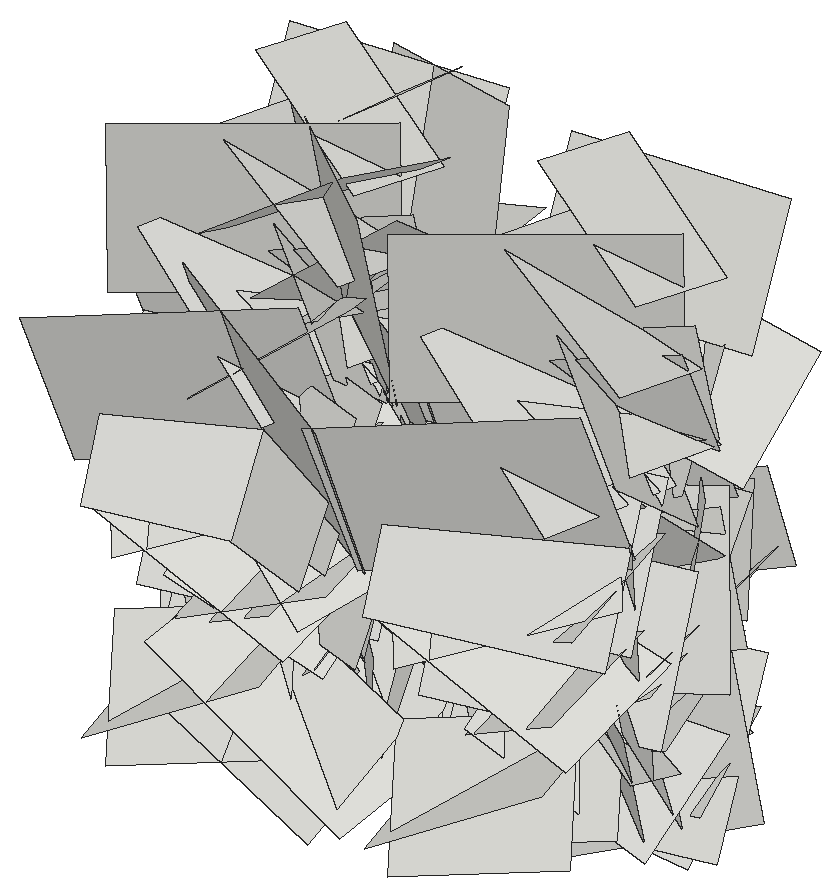
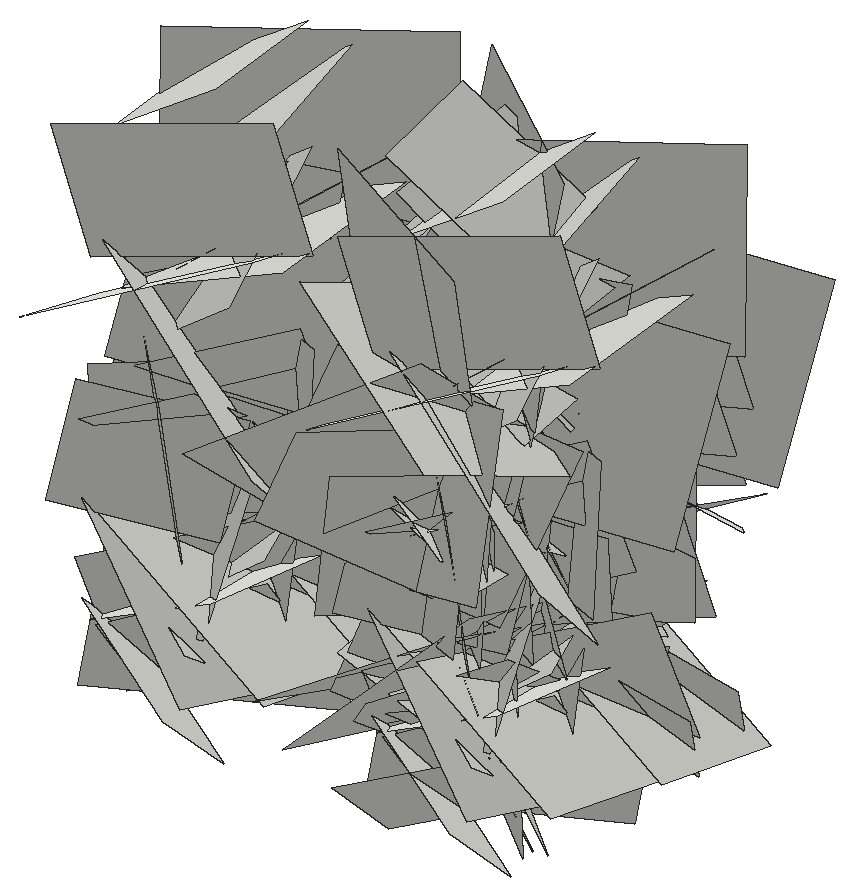
# SketchUp Ruby script. Lengths in inches.
U = 1.inch
M = Sketchup.active_model
def pt(a) = Geom::Point3d.new(a.map { |v| v * U })
def face(e, loops, mat)
  f = e.add_face(loops[0].map { |a| pt(a) })
  loops[1..].each { |l| e.add_face(l.map { |a| pt(a) }).erase! }
  f.material = f.back_material = mat if mat
  f
end
# faces: each face lists its corners as indices into pts; further lists are holes
def faces(e, pts, list, mat = nil) = list.each { |f| face(e, (f[0].is_a?(Array) ? f : [f]).map { |l| l.map { |i| pts[i] } }, mat) }
# xy, xz, yz: faces in a plane at the given z, y or x. An outline is a flat list of corners, or four numbers for a rectangle; further outlines are holes
def ring(l) = l.size == 4 ? [[l[0], l[1]], [l[2], l[1]], [l[2], l[3]], [l[0], l[3]]] : l.each_slice(2).to_a
def flat(e, list, mat, &to3) = list.each { |f| face(e, (f[0].is_a?(Array) ? f : [f]).map { |l| ring(l).map { |u, v| to3.(u, v) } }, mat) }
def xy(e, z, list, mat = nil) = flat(e, list, mat) { |x, y| [x, y, z] }
def xz(e, y, list, mat = nil) = flat(e, list, mat) { |x, z| [x, y, z] }
def yz(e, x, list, mat = nil) = flat(e, list, mat) { |y, z| [x, y, z] }
def lines(e, pts, list) = list.each { |a, b| e.add_line(pt(pts[a]), pt(pts[b])) }
# prism: a flat outline (further loops are holes) pulled along v
def prism(e, loops, v, mat = nil)
  f = face(e, loops, mat); d = Geom::Vector3d.new(v.map { |x| x * U })
  f.pushpull(f.normal.samedirection?(d) ? d.length : -d.length)
end
def box(e, o, s, mat = nil) = prism(e, [[o, [o[0] + s[0], o[1], o[2]], [o[0] + s[0], o[1] + s[1], o[2]], [o[0], o[1] + s[1], o[2]]]], [0, 0, s[2]], mat)
def at(x, y, z, deg = 0) = Geom::Transformation.translation(pt([x, y, z])) * Geom::Transformation.rotation(ORIGIN, Z_AXIS, deg.degrees)
def axes(o, x, y, z) = Geom::Transformation.new([*x, 0, *y, 0, *z, 0, *pt(o).to_a, 1])
def part(name) = M.definitions.add(name)
# library, detail: a bought-in or finely detailed component or shape, given as its bounding box
def library(name, o, s) = part(name).tap { |d| box(d.entities, o, s) }
def detail(e, o, s) = box(e.add_group.entities, o, s)
def put(e, d, t, mat = nil) = e.add_instance(d, t).tap { |i| i.material = mat if mat }
def group(e, t, mat = nil) = e.add_group.tap { |g| g.transformation = t; g.material = mat if mat }.entities
root = M.entities
c1 = part("Component\#6")
p = [[0.01,0,0],[0,3.24,4.54],[4.32,3.24,4.54],[4.33,0,0]]
faces(c1.entities,p,[[0,1,2,3]])
put(root,c1,axes([18.5,124,36.29],[0.02149,0.52903,-1.24729],[-0.2007,-1.23408,-0.5265],[-1.42204,0.18216,0.05546]))
put(root,c1,axes([14.53,124,36.29],[-0.02149,0.52903,-1.24729],[0.2007,-1.23408,-0.5265],[1.42204,0.18216,0.05546]))
put(root,c1,axes([28.31,124,36.29],[0.02149,0.52903,-1.24729],[-0.2007,-1.23408,-0.5265],[-1.42204,0.18216,0.05546]))
put(root,c1,axes([18.56,123.49,22.43],[-0.36857,0.54861,0.76203],[-0.54406,0.56941,-0.64413],[-0.83345,-0.61431,0.08349]))
put(root,c1,axes([14.48,123.49,22.43],[0.36857,0.54861,0.76203],[0.54406,0.56941,-0.64413],[0.83345,-0.61431,0.08349]))
put(root,c1,axes([28.36,123.49,22.43],[-0.36857,0.54861,0.76203],[-0.54406,0.56941,-0.64413],[-0.83345,-0.61431,0.08349]))
put(root,c1,axes([18.5,126.73,32.74],[0.07983,-0.47542,-1.06148],[-0.1788,-1.05692,0.46141],[-1.21984,0.1238,-0.1371]))
put(root,c1,axes([14.53,126.73,32.74],[-0.07983,-0.47542,-1.06148],[0.1788,-1.05692,0.46141],[1.21984,0.1238,-0.1371]))
put(root,c1,axes([28.31,126.73,32.74],[0.07983,-0.47542,-1.06148],[-0.1788,-1.05692,0.46141],[-1.21984,0.1238,-0.1371]))
put(root,c1,axes([18.5,122.33,25.2],[-0.14417,1.26196,0.33106],[-0.05821,0.32703,-1.26913],[-1.38172,-0.14545,0.01892]))
put(root,c1,axes([14.53,122.33,25.2],[0.14417,1.26196,0.33106],[0.05821,0.32703,-1.26913],[1.38172,-0.14545,0.01892]))
put(root,c1,axes([28.31,122.33,25.2],[-0.14417,1.26196,0.33106],[-0.05821,0.32703,-1.26913],[-1.38172,-0.14545,0.01892]))
put(root,c1,axes([18.5,127.85,32.74],[0.07983,-0.47542,-1.06148],[-0.1788,-1.05692,0.46141],[-1.21984,0.1238,-0.1371]))
put(root,c1,axes([14.53,127.85,32.74],[-0.07983,-0.47542,-1.06148],[0.1788,-1.05692,0.46141],[1.21984,0.1238,-0.1371]))
put(root,c1,axes([28.31,127.85,32.74],[0.07983,-0.47542,-1.06148],[-0.1788,-1.05692,0.46141],[-1.21984,0.1238,-0.1371]))
put(root,c1,axes([14.53,128.39,27.01],[0.01413,-1.13969,-0.35832],[0.11214,-0.35581,1.13564],[1.2614,0.04439,-0.09695]))
put(root,c1,axes([18.5,128.39,27.01],[-0.01413,-1.13969,-0.35832],[-0.11214,-0.35581,1.13564],[-1.2614,0.04439,-0.09695]))
put(root,c1,axes([28.31,128.39,27.01],[-0.01413,-1.13969,-0.35832],[-0.11214,-0.35581,1.13564],[-1.2614,0.04439,-0.09695]))
put(root,c1,axes([19.22,124.93,30.08],[-0.69154,0.83647,0.57299],[-0.50453,0.34895,-1.05134],[-0.94895,-0.79509,0.14141]))
put(root,c1,axes([13.82,124.93,30.08],[0.69154,0.83647,0.57299],[0.50453,0.34895,-1.05134],[0.94895,-0.79509,0.14141]))
put(root,c1,axes([29.02,124.93,30.08],[-0.69154,0.83647,0.57299],[-0.50453,0.34895,-1.05134],[-0.94895,-0.79509,0.14141]))
put(root,c1,axes([14.53,128.06,26.23],[-0.10092,-0.80547,-0.37503],[-0.00485,-0.37672,0.81027],[0.94179,-0.08825,-0.03602]))
put(root,c1,axes([24.34,128.06,26.23],[-0.10092,-0.80547,-0.37503],[-0.00485,-0.37672,0.81027],[0.94179,-0.08825,-0.03602]))
put(root,c1,axes([18.5,128.06,26.23],[0.10092,-0.80547,-0.37503],[0.00485,-0.37672,0.81027],[-0.94179,-0.08825,-0.03602]))
put(root,c1,axes([18.5,128.2,32.33],[-0.15852,-1.12421,0.05612],[0.12401,0.04078,1.12872],[-1.18668,0.15444,0.11046]))
put(root,c1,axes([14.53,128.2,32.33],[0.15852,-1.12421,0.05612],[-0.12401,0.04078,1.12872],[1.18668,0.15444,0.11046]))
put(root,c1,axes([28.31,128.2,32.33],[-0.15852,-1.12421,0.05612],[0.12401,0.04078,1.12872],[-1.18668,0.15444,0.11046]))
put(root,c1,axes([18.56,125.55,22.43],[-0.36857,0.54861,0.76203],[-0.54406,0.56941,-0.64413],[-0.83345,-0.61431,0.08349]))
put(root,c1,axes([14.48,125.55,22.43],[0.36857,0.54861,0.76203],[0.54406,0.56941,-0.64413],[0.83345,-0.61431,0.08349]))
put(root,c1,axes([28.36,125.55,22.43],[-0.36857,0.54861,0.76203],[-0.54406,0.56941,-0.64413],[-0.83345,-0.61431,0.08349]))
put(root,c1,axes([14.53,129.13,29.07],[-0.11411,-0.79222,-0.47459],[-0.01099,-0.47673,0.79815],[0.97884,-0.0977,-0.04636]))
put(root,c1,axes([24.34,129.13,29.07],[-0.11411,-0.79222,-0.47459],[-0.01099,-0.47673,0.79815],[0.97884,-0.0977,-0.04636]))
put(root,c1,axes([18.5,129.13,29.07],[0.11411,-0.79222,-0.47459],[0.01099,-0.47673,0.79815],[-0.97884,-0.0977,-0.04636]))
put(root,c1,axes([14.53,128.47,40.0625],[0.15368,0.21217,-1.35934],[-0.08132,-1.3635,-0.221],[1.45608,-0.09854,0.13113]))
put(root,c1,axes([18.5,128.47,40.0625],[-0.15368,0.21217,-1.35934],[0.08132,-1.3635,-0.221],[-1.45608,-0.09854,0.13113]))
put(root,c1,axes([28.31,128.47,40.0625],[-0.15368,0.21217,-1.35934],[0.08132,-1.3635,-0.221],[-1.45608,-0.09854,0.13113]))
put(root,c1,axes([14.53,129.14,29.25],[-0.07983,-0.47542,-1.06148],[0.1788,-1.05692,0.46141],[1.21984,0.1238,-0.1371]))
put(root,c1,axes([18.5,129.14,29.25],[0.07983,-0.47542,-1.06148],[-0.1788,-1.05692,0.46141],[-1.21984,0.1238,-0.1371]))
put(root,c1,axes([28.31,129.14,29.25],[0.07983,-0.47542,-1.06148],[-0.1788,-1.05692,0.46141],[-1.21984,0.1238,-0.1371]))
put(root,c1,axes([18.5,126.77,21.87],[0.10992,-0.34124,0.92241],[-0.05569,0.92428,0.34784],[-1.04103,-0.08548,0.07879]))
put(root,c1,axes([14.53,126.77,21.87],[-0.10992,-0.34124,0.92241],[0.05569,0.92428,0.34784],[1.04103,-0.08548,0.07879]))
put(root,c1,axes([28.31,126.77,21.87],[0.10992,-0.34124,0.92241],[-0.05569,0.92428,0.34784],[-1.04103,-0.08548,0.07879]))
put(root,c1,axes([14.53,129.34,35.47],[-0.09463,-0.94647,0.23979],[-0.00571,0.24126,0.95028],[1.03494,-0.08521,0.02717]))
put(root,c1,axes([18.5,129.34,35.47],[0.09463,-0.94647,0.23979],[0.00571,0.24126,0.95028],[-1.03494,-0.08521,0.02717]))
put(root,c1,axes([28.31,129.34,35.47],[0.09463,-0.94647,0.23979],[0.00571,0.24126,0.95028],[-1.03494,-0.08521,0.02717]))
put(root,c1,axes([14.53,130.61,23.63],[-0.04049,-0.92661,-0.53015],[-0.18829,-0.51758,0.91743],[1.11583,-0.12096,0.13557]))
put(root,c1,axes([18.5,130.61,23.63],[0.04049,-0.92661,-0.53015],[0.18829,-0.51758,0.91743],[-1.11583,-0.12096,0.13557]))
put(root,c1,axes([28.31,130.61,23.63],[0.04049,-0.92661,-0.53015],[0.18829,-0.51758,0.91743],[-1.11583,-0.12096,0.13557]))
put(root,c1,axes([18.5,126.5625,26.98],[0.04661,-0.13743,1.04442],[-0.16266,1.03335,0.14244],[-1.10472,-0.15795,0.02309]))
put(root,c1,axes([14.53,126.5625,26.98],[-0.04661,-0.13743,1.04442],[0.16266,1.03335,0.14244],[1.10472,-0.15795,0.02309]))
put(root,c1,axes([28.31,126.5625,26.98],[0.04661,-0.13743,1.04442],[-0.16266,1.03335,0.14244],[-1.10472,-0.15795,0.02309]))
put(root,c1,axes([14.53,128.14,26.625],[-0.13018,-0.67547,0.62862],[-0.07474,0.63918,0.67304],[0.97523,-0.04118,0.13549]))
put(root,c1,axes([24.34,128.14,26.625],[-0.13018,-0.67547,0.62862],[-0.07474,0.63918,0.67304],[0.97523,-0.04118,0.13549]))
put(root,c1,axes([18.5,128.14,26.625],[0.13018,-0.67547,0.62862],[0.07474,0.63918,0.67304],[-0.97523,-0.04118,0.13549]))
put(root,c1,axes([14.53,130.48,31.34],[-0.20009,-0.24055,-1.32848],[-0.01815,-1.34087,0.24522],[1.43098,-0.05064,-0.18264]))
put(root,c1,axes([18.5,130.48,31.34],[0.20009,-0.24055,-1.32848],[0.01815,-1.34087,0.24522],[-1.43098,-0.05064,-0.18264]))
put(root,c1,axes([28.31,130.48,31.34],[0.20009,-0.24055,-1.32848],[0.01815,-1.34087,0.24522],[-1.43098,-0.05064,-0.18264]))
put(root,c1,axes([14.53,126.29,27.49],[-0.18614,0.86586,-0.34095],[-0.04817,-0.35453,-0.87695],[0.98523,0.14625,-0.10729]))
put(root,c1,axes([18.5,126.29,27.49],[0.18614,0.86586,-0.34095],[0.04817,-0.35453,-0.87695],[-0.98523,0.14625,-0.10729]))
put(root,c1,axes([24.34,126.29,27.49],[-0.18614,0.86586,-0.34095],[-0.04817,-0.35453,-0.87695],[0.98523,0.14625,-0.10729]))
put(root,c1,axes([14.53,130.13,32.75],[0.05656,-1.14018,0.16245],[0.17438,0.16851,1.12862],[1.20828,0.02906,-0.17049]))
put(root,c1,axes([18.5,130.13,32.75],[-0.05656,-1.14018,0.16245],[-0.17438,0.16851,1.12862],[-1.20828,0.02906,-0.17049]))
put(root,c1,axes([28.31,130.13,32.75],[-0.05656,-1.14018,0.16245],[-0.17438,0.16851,1.12862],[-1.20828,0.02906,-0.17049]))
put(root,c1,axes([18.5,128.45,36.29],[0.02149,0.52903,-1.24729],[-0.2007,-1.23408,-0.5265],[-1.42204,0.18216,0.05546]))
put(root,c1,axes([14.53,128.45,36.29],[-0.02149,0.52903,-1.24729],[0.2007,-1.23408,-0.5265],[1.42204,0.18216,0.05546]))
put(root,c1,axes([28.31,128.45,36.29],[0.02149,0.52903,-1.24729],[-0.2007,-1.23408,-0.5265],[-1.42204,0.18216,0.05546]))
put(root,c1,axes([14.53,129.02,36.97],[-0.03047,0.19902,-0.90037],[0.05941,-0.89877,-0.20045],[0.97562,0.06094,-0.01591]))
put(root,c1,axes([18.5,129.02,36.97],[0.03047,0.19902,-0.90037],[-0.05941,-0.89877,-0.20045],[-0.97562,0.06094,-0.01591]))
put(root,c1,axes([28.31,129.02,36.97],[0.03047,0.19902,-0.90037],[-0.05941,-0.89877,-0.20045],[-0.97562,0.06094,-0.01591]))
put(root,c1,axes([18.5,130.54,26.21],[0.16316,0.13144,-1.2549],[0.21583,-1.25022,-0.10597],[-1.31994,-0.18819,-0.17245]))
put(root,c1,axes([14.53,130.54,26.21],[-0.16316,0.13144,-1.2549],[-0.21583,-1.25022,-0.10597],[1.31994,-0.18819,-0.17245]))
put(root,c1,axes([28.31,130.54,26.21],[0.16316,0.13144,-1.2549],[0.21583,-1.25022,-0.10597],[-1.31994,-0.18819,-0.17245]))
put(root,c1,axes([14.53,129.15,30.625],[-0.089,-0.93417,0.70597],[-0.20388,0.70917,0.91554],[1.22433,0.05019,0.20378]))
put(root,c1,axes([18.5,129.15,30.625],[0.089,-0.93417,0.70597],[0.20388,0.70917,0.91554],[-1.22433,0.05019,0.20378]))
put(root,c1,axes([28.31,129.15,30.625],[0.089,-0.93417,0.70597],[0.20388,0.70917,0.91554],[-1.22433,0.05019,0.20378]))
put(root,c1,axes([14.53,132.16,25.41],[-0.07094,-0.60211,-1.2376],[-0.1162,-1.23279,0.6057],[1.45423,-0.12788,-0.01197]))
put(root,c1,axes([18.5,132.16,25.41],[0.07094,-0.60211,-1.2376],[0.1162,-1.23279,0.6057],[-1.45423,-0.12788,-0.01197]))
put(root,c1,axes([28.31,132.16,25.41],[0.07094,-0.60211,-1.2376],[0.1162,-1.23279,0.6057],[-1.45423,-0.12788,-0.01197]))
put(root,c1,axes([14.53,130.09,30.86],[-0.13772,0.10296,-1.023],[-0.01142,-1.03121,-0.10242],[1.08979,0.0022,-0.13035]))
put(root,c1,axes([18.5,130.09,30.86],[0.13772,0.10296,-1.023],[0.01142,-1.03121,-0.10242],[-1.08979,0.0022,-0.13035]))
put(root,c1,axes([28.31,130.09,30.86],[0.13772,0.10296,-1.023],[0.01142,-1.03121,-0.10242],[-1.08979,0.0022,-0.13035]))
put(root,c1,axes([14.53,130.39,37.85],[0.05885,-0.83818,0.13983],[-0.03078,0.13818,0.83979],[0.90022,0.05952,0.01957]))
put(root,c1,axes([18.5,130.39,37.85],[-0.05885,-0.83818,0.13983],[0.03078,0.13818,0.83979],[-0.90022,0.05952,0.01957]))
put(root,c1,axes([28.31,130.39,37.85],[-0.05885,-0.83818,0.13983],[0.03078,0.13818,0.83979],[-0.90022,0.05952,0.01957]))
put(root,c1,axes([14.53,128.44,21.53],[-0.07533,-0.68545,1.00594],[-0.30491,0.98857,0.65329],[1.25377,0.19923,0.21932]))
put(root,c1,axes([18.5,128.44,21.53],[0.07533,-0.68545,1.00594],[0.30491,0.98857,0.65329],[-1.25377,0.19923,0.21932]))
put(root,c1,axes([28.31,128.44,21.53],[0.07533,-0.68545,1.00594],[0.30491,0.98857,0.65329],[-1.25377,0.19923,0.21932]))
put(root,c1,axes([14.53,131.26,22.93],[0.10206,-0.4663,-0.72841],[0.02316,-0.73136,0.47108],[0.91647,0.07041,0.06921]))
put(root,c1,axes([18.5,131.26,22.93],[-0.10206,-0.4663,-0.72841],[-0.02316,-0.73136,0.47108],[-0.91647,0.07041,0.06921]))
put(root,c1,axes([28.31,131.26,22.93],[-0.10206,-0.4663,-0.72841],[-0.02316,-0.73136,0.47108],[-0.91647,0.07041,0.06921]))
put(root,c1,axes([14.53,131.47,30.67],[0.19347,-0.24403,-0.96391],[-0.05093,-0.98104,0.23927],[1.05275,-0.00261,0.18872]))
put(root,c1,axes([18.5,131.47,30.67],[-0.19347,-0.24403,-0.96391],[0.05093,-0.98104,0.23927],[-1.05275,-0.00261,0.18872]))
put(root,c1,axes([28.31,131.47,30.67],[-0.19347,-0.24403,-0.96391],[0.05093,-0.98104,0.23927],[-1.05275,-0.00261,0.18872]))
put(root,c1,axes([14.53,131.58,31.0625],[0.07279,0.01987,-1.05868],[-0.10279,-1.05633,-0.02611],[1.11768,-0.09844,0.06655]))
put(root,c1,axes([18.5,131.58,31.0625],[-0.07279,0.01987,-1.05868],[0.10279,-1.05633,-0.02611],[-1.11768,-0.09844,0.06655]))
put(root,c1,axes([28.31,131.58,31.0625],[-0.07279,0.01987,-1.05868],[0.10279,-1.05633,-0.02611],[-1.11768,-0.09844,0.06655]))
put(root,c1,axes([14.53,131.52,23.18],[0.15485,-0.9106,-0.00305],[0.11373,0.01414,0.91588],[0.95852,0.14543,-0.10818]))
put(root,c1,axes([18.5,131.52,23.18],[-0.15485,-0.9106,-0.00305],[-0.11373,0.01414,0.91588],[-0.95852,0.14543,-0.10818]))
put(root,c1,axes([28.31,131.52,23.18],[-0.15485,-0.9106,-0.00305],[-0.11373,0.01414,0.91588],[-0.95852,0.14543,-0.10818]))
put(root,c1,axes([18.5,127.05,26.22],[-0.14417,1.26196,0.33106],[-0.05821,0.32703,-1.26913],[-1.38172,-0.14545,0.01892]))
put(root,c1,axes([14.53,127.05,26.22],[0.14417,1.26196,0.33106],[0.05821,0.32703,-1.26913],[1.38172,-0.14545,0.01892]))
put(root,c1,axes([28.31,127.05,26.22],[-0.14417,1.26196,0.33106],[-0.05821,0.32703,-1.26913],[-1.38172,-0.14545,0.01892]))
put(root,c1,axes([18.5,127.73,24.28],[0.02979,0.75993,0.53946],[0.00151,0.53967,-0.7603],[-0.98786,0.02374,0.0151]))
put(root,c1,axes([14.53,127.73,24.28],[-0.02979,0.75993,0.53946],[-0.00151,0.53967,-0.7603],[0.98786,0.02374,0.0151]))
put(root,c1,axes([28.31,127.73,24.28],[0.02979,0.75993,0.53946],[0.00151,0.53967,-0.7603],[-0.98786,0.02374,0.0151]))
put(root,c1,axes([18.5,127.1,26.99],[0.01407,1.25738,0.35681],[0.29384,0.346,-1.2296],[-1.35392,0.08816,-0.26315]))
put(root,c1,axes([14.53,127.1,26.99],[-0.01407,1.25738,0.35681],[-0.29384,0.346,-1.2296],[1.35392,0.08816,-0.26315]))
put(root,c1,axes([28.31,127.1,26.99],[0.01407,1.25738,0.35681],[0.29384,0.346,-1.2296],[-1.35392,0.08816,-0.26315]))
put(root,c1,axes([14.53,129.03,31.05],[0.04043,0.74356,0.04678],[0.07255,0.04314,-0.74161],[0.78639,-0.04221,0.06601]))
put(root,c1,axes([18.5,129.03,31.05],[-0.04043,0.74356,0.04678],[-0.07255,0.04314,-0.74161],[-0.78639,-0.04221,0.06601]))
put(root,c1,axes([18.5,134.48,33.76],[0.26334,-1.11466,-0.41014],[-0.1173,-0.43892,1.12584],[-1.25351,-0.19309,-0.19152]))
put(root,c1,axes([14.53,134.48,33.76],[-0.26334,-1.11466,-0.41014],[0.1173,-0.43892,1.12584],[1.25351,-0.19309,-0.19152]))
put(root,c1,axes([28.31,134.48,33.76],[0.26334,-1.11466,-0.41014],[-0.1173,-0.43892,1.12584],[-1.25351,-0.19309,-0.19152]))
put(root,c1,axes([14.53,133.52,31.89],[-0.15087,-0.04242,-1.05475],[-0.23169,-1.04005,0.07132],[1.09469,-0.22597,-0.13027]))
put(root,c1,axes([18.5,133.52,31.89],[0.15087,-0.04242,-1.05475],[0.23169,-1.04005,0.07132],[-1.09469,-0.22597,-0.13027]))
put(root,c1,axes([24.34,133.52,31.89],[-0.15087,-0.04242,-1.05475],[-0.23169,-1.04005,0.07132],[1.09469,-0.22597,-0.13027]))
put(root,c1,axes([14.53,129.22,21.54],[-0.01805,0.58513,0.55019],[0.06792,0.54955,-0.58247],[0.84865,-0.03153,0.05832]))
put(root,c1,axes([18.5,129.22,21.54],[0.01805,0.58513,0.55019],[-0.06792,0.54955,-0.58247],[-0.84865,-0.03153,0.05832]))
put(root,c1,axes([28.31,129.22,21.54],[0.01805,0.58513,0.55019],[-0.06792,0.54955,-0.58247],[-0.84865,-0.03153,0.05832]))
put(root,c1,axes([14.53,129.75,30.06],[0.01937,0.49926,0.36665],[0.0577,0.36409,-0.4985],[0.65405,-0.04691,0.03312]))
put(root,c1,axes([24.34,129.75,30.06],[0.01937,0.49926,0.36665],[0.0577,0.36409,-0.4985],[0.65405,-0.04691,0.03312]))
put(root,c1,axes([18.5,129.75,30.06],[-0.01937,0.49926,0.36665],[-0.0577,0.36409,-0.4985],[-0.65405,-0.04691,0.03312]))
put(root,c1,axes([18.5,133.17,39.1],[-0.0845,-0.28698,-1.03421],[-0.22383,-1.0126,0.29726],[-1.11545,0.22493,0.0187]))
put(root,c1,axes([14.53,133.17,39.1],[0.0845,-0.28698,-1.03421],[0.22383,-1.0126,0.29726],[1.11545,0.22493,0.0187]))
put(root,c1,axes([28.31,133.17,39.1],[-0.0845,-0.28698,-1.03421],[-0.22383,-1.0126,0.29726],[-1.11545,0.22493,0.0187]))
put(root,c1,axes([14.53,128.43,31.91],[0.33386,1.00192,0.91989],[0.02581,0.93993,-1.03208],[1.44154,-0.24887,-0.19457]))
put(root,c1,axes([18.5,128.43,31.91],[-0.33386,1.00192,0.91989],[-0.02581,0.93993,-1.03208],[-1.44154,-0.24887,-0.19457]))
put(root,c1,axes([28.31,128.43,31.91],[-0.33386,1.00192,0.91989],[-0.02581,0.93993,-1.03208],[-1.44154,-0.24887,-0.19457]))
put(root,c1,axes([14.53,130.92,26.67],[-0.06799,-0.20959,0.7931],[0.02884,0.79454,0.21217],[0.86907,-0.04277,0.05501]))
put(root,c1,axes([24.34,130.92,26.67],[-0.06799,-0.20959,0.7931],[0.02884,0.79454,0.21217],[0.86907,-0.04277,0.05501]))
put(root,c1,axes([18.5,130.92,26.67],[0.06799,-0.20959,0.7931],[-0.02884,0.79454,0.21217],[-0.86907,-0.04277,0.05501]))
put(root,c1,axes([18.5,131.21,27.63],[0.2234,-0.54463,1.08834],[0.02633,1.10624,0.54877],[-1.28976,-0.07175,0.19972]))
put(root,c1,axes([14.53,131.21,27.63],[-0.2234,-0.54463,1.08834],[-0.02633,1.10624,0.54877],[1.28976,-0.07175,0.19972]))
